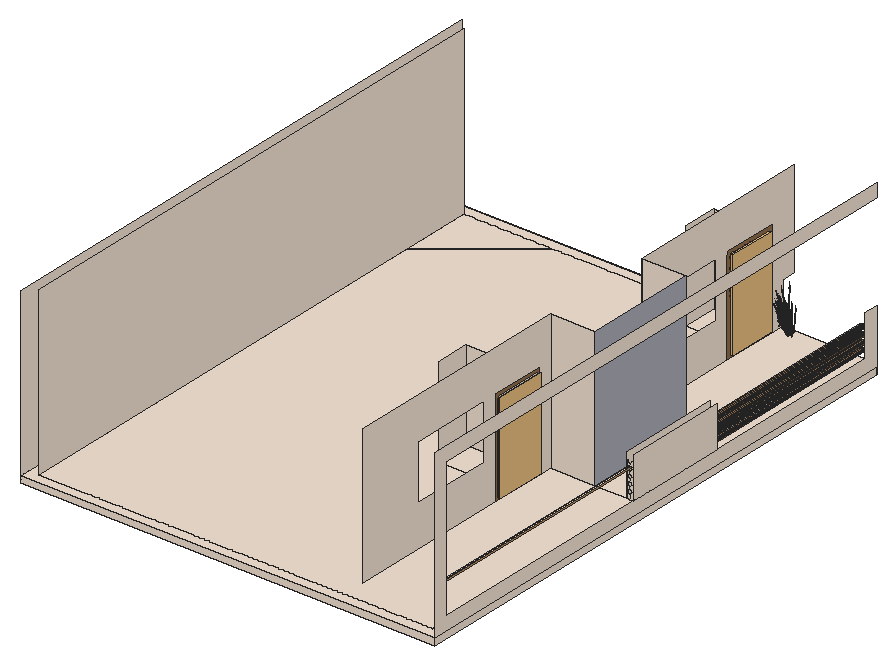
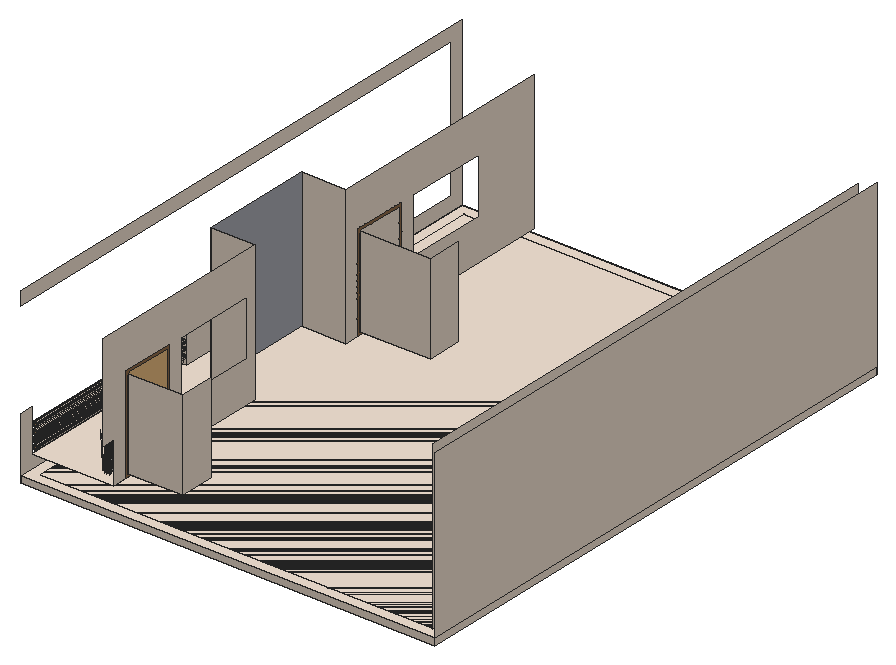
# SketchUp Ruby script. Lengths in inches.
U = 1.inch
M = Sketchup.active_model
def pt(a) = Geom::Point3d.new(a.map { |v| v * U })
def face(e, loops, mat)
  f = e.add_face(loops[0].map { |a| pt(a) })
  loops[1..].each { |l| e.add_face(l.map { |a| pt(a) }).erase! }
  f.material = f.back_material = mat if mat
  f
end
# faces: each face lists its corners as indices into pts; further lists are holes
def faces(e, pts, list, mat = nil) = list.each { |f| face(e, (f[0].is_a?(Array) ? f : [f]).map { |l| l.map { |i| pts[i] } }, mat) }
# xy, xz, yz: faces in a plane at the given z, y or x. An outline is a flat list of corners, or four numbers for a rectangle; further outlines are holes
def ring(l) = l.size == 4 ? [[l[0], l[1]], [l[2], l[1]], [l[2], l[3]], [l[0], l[3]]] : l.each_slice(2).to_a
def flat(e, list, mat, &to3) = list.each { |f| face(e, (f[0].is_a?(Array) ? f : [f]).map { |l| ring(l).map { |u, v| to3.(u, v) } }, mat) }
def xy(e, z, list, mat = nil) = flat(e, list, mat) { |x, y| [x, y, z] }
def xz(e, y, list, mat = nil) = flat(e, list, mat) { |x, z| [x, y, z] }
def yz(e, x, list, mat = nil) = flat(e, list, mat) { |y, z| [x, y, z] }
def lines(e, pts, list) = list.each { |a, b| e.add_line(pt(pts[a]), pt(pts[b])) }
# prism: a flat outline (further loops are holes) pulled along v
def prism(e, loops, v, mat = nil)
  f = face(e, loops, mat); d = Geom::Vector3d.new(v.map { |x| x * U })
  f.pushpull(f.normal.samedirection?(d) ? d.length : -d.length)
end
def box(e, o, s, mat = nil) = prism(e, [[o, [o[0] + s[0], o[1], o[2]], [o[0] + s[0], o[1] + s[1], o[2]], [o[0], o[1] + s[1], o[2]]]], [0, 0, s[2]], mat)
def at(x, y, z, deg = 0) = Geom::Transformation.translation(pt([x, y, z])) * Geom::Transformation.rotation(ORIGIN, Z_AXIS, deg.degrees)
def axes(o, x, y, z) = Geom::Transformation.new([*x, 0, *y, 0, *z, 0, *pt(o).to_a, 1])
def part(name) = M.definitions.add(name)
# library, detail: a bought-in or finely detailed component or shape, given as its bounding box
def library(name, o, s) = part(name).tap { |d| box(d.entities, o, s) }
def detail(e, o, s) = box(e.add_group.entities, o, s)
def put(e, d, t, mat = nil) = e.add_instance(d, t).tap { |i| i.material = mat if mat }
def group(e, t, mat = nil) = e.add_group.tap { |g| g.transformation = t; g.material = mat if mat }.entities
root = M.entities
M.materials.add("C01_Vanilla_Cream").color = [244, 228, 212]
M.materials.add("LightPink_Translucent").color = [144, 107, 117]
M.materials["LightPink_Translucent"].alpha = 0.75
M.materials.add("Marble_20_1K").color = [172, 173, 182]
M.materials.add("Wood_Floor_01_1K").color = [146, 111, 76]
c1 = library("porta+4",[0.2,-5.42,1.33],[46.55,4.72,83.21])
c2 = part("Group\#10")
box(c2.entities,[0,0,0],[360,480,6])
c3 = part("blade")
p = [[2.15,0.21,22],[0,0.17,0],[0.09,0.45,0],[2.18,0.31,22],[2.29,0.31,22],[0.38,0.45,0],
  [2.48,0.24,33],[2.49,0.24,33],[2.48,0.22,33]]
faces(c3.entities,p,[[0,1,2,3],[4,5,2,3],[6,3,4,7],[8,0,3,6]])
c4 = part("seeds")
p = [[0.3,-0.1,1.38],[-0.01,-0.03,1.59],[-0.01,-0.03,0.03],[0.14,-0.07,-0.07],[0.29,-0.03,3],[0.15,0.01,3.11]]
faces(c4.entities,p,[[0,1,2,3],[1,0,4,5]],"LightPink_Translucent")
c5 = part("blade with seeds")
put(c5.entities,c3,at(0,0,0))
put(c5.entities,c4,axes([2.4,0.25,30.99],[1.5799,-0.05474,1.17369],[-0.12525,1.92788,0.29478],[-0.07173,-0.02425,1.56792]))
xy(root,444,[[[0,0,360,480],[9,9,351,471]]],"C01_Vanilla_Cream")
xy(root,450,[[[0,0,360,480],[9,9,351,471]],[9,9,351,471]],"C01_Vanilla_Cream")
xy(root,462,[[326.85,216,354,216,354,306.76,360,306.76,360,468,288,468,288,314.71,326.85,314.71],[354,216,360,306.76]],"C01_Vanilla_Cream")
xy(root,465,[[226.53,171,288,201],[240,423,288,453]],"C01_Vanilla_Cream")
xz(root,201,[[226.53,465,288,543]],"C01_Vanilla_Cream")
xz(root,216,[[288,462,326.85,582],[354,462,357,462,357,466,356.48,466.07,356,466.27,355.59,466.59,355.27,467,355.07,467.48,355,468,354,468],[357,462,360,462,360,468,359,468,358.93,467.48,358.73,467,358.41,466.59,358,466.27,357.52,466.07,357,466],[354,468,355,468,355.07,468.52,355.27,469,355.59,469.41,356,469.73,356.48,469.93,357,470,357,472,356.48,472.07,356,472.27,355.59,472.59,355.27,473,355.07,473.48,355,474,354,474],[359,468,360,468,360,474,359,474,358.93,473.48,358.73,473,358.41,472.59,358,472.27,357.52,472.07,357,472,357,470,357.52,469.93,358,469.73,358.41,469.41,358.73,469,358.93,468.52],
  [354,474,355,474,355.07,474.52,355.27,475,355.59,475.41,356,475.73,356.48,475.93,357,476,357,478,356.48,478.07,356,478.27,355.59,478.59,355.27,479,355.07,479.48,355,480,354,480],[359,474,360,474,360,480,359,480,358.93,479.48,358.73,479,358.41,478.59,358,478.27,357.52,478.07,357,478,357,476,357.52,475.93,358,475.73,358.41,475.41,358.73,475,358.93,474.52],[354,480,355,480,355.07,480.52,355.27,481,355.59,481.41,356,481.73,356.48,481.93,357,482,357,484,356.48,484.07,356,484.27,355.59,484.59,355.27,485,355.07,485.48,355,486,354,486],[359,480,360,480,360,486,359,486,358.93,485.48,358.73,485,358.41,484.59,358,484.27,357.52,484.07,357,484,357,482,357.52,481.93,358,481.73,358.41,481.41,358.73,481,358.93,480.52],[354,486,355,486,355.07,486.52,355.27,487,355.59,487.41,356,487.73,356.48,487.93,357,488,357,490,356.48,490.07,356,490.27,355.59,490.59,355.27,491,355.07,491.48,355,492,354,492],
  [359,486,360,486,360,492,359,492,358.93,491.48,358.73,491,358.41,490.59,358,490.27,357.52,490.07,357,490,357,488,357.52,487.93,358,487.73,358.41,487.41,358.73,487,358.93,486.52]],"C01_Vanilla_Cream")
xz(root,306.76,[[354,462,354,468,355,468,355.07,467.48,355.27,467,355.59,466.59,356,466.27,356.48,466.07,357,466,357,462],[357,462,357,466,357.52,466.07,358,466.27,358.41,466.59,358.73,467,358.93,467.48,359,468,360,468,360,462],[354,468,354,474,355,474,355.07,473.48,355.27,473,355.59,472.59,356,472.27,356.48,472.07,357,472,357,470,356.48,469.93,356,469.73,355.59,469.41,355.27,469,355.07,468.52,355,468],[359,468,358.93,468.52,358.73,469,358.41,469.41,358,469.73,357.52,469.93,357,470,357,472,357.52,472.07,358,472.27,358.41,472.59,358.73,473,358.93,473.48,359,474,360,474,360,468],[354,474,354,480,355,480,355.07,479.48,355.27,479,355.59,478.59,356,478.27,356.48,478.07,357,478,357,476,356.48,475.93,356,475.73,355.59,475.41,355.27,475,355.07,474.52,355,474],
  [359,474,358.93,474.52,358.73,475,358.41,475.41,358,475.73,357.52,475.93,357,476,357,478,357.52,478.07,358,478.27,358.41,478.59,358.73,479,358.93,479.48,359,480,360,480,360,474],[354,480,354,486,355,486,355.07,485.48,355.27,485,355.59,484.59,356,484.27,356.48,484.07,357,484,357,482,356.48,481.93,356,481.73,355.59,481.41,355.27,481,355.07,480.52,355,480],[359,480,358.93,480.52,358.73,481,358.41,481.41,358,481.73,357.52,481.93,357,482,357,484,357.52,484.07,358,484.27,358.41,484.59,358.73,485,358.93,485.48,359,486,360,486,360,480],[354,486,354,492,355,492,355.07,491.48,355.27,491,355.59,490.59,356,490.27,356.48,490.07,357,490,357,488,356.48,487.93,356,487.73,355.59,487.41,355.27,487,355.07,486.52,355,486],[359,486,358.93,486.52,358.73,487,358.41,487.41,358,487.73,357.52,487.93,357,488,357,490,357.52,490.07,358,490.27,358.41,490.59,358.73,491,358.93,491.48,359,492,360,492,360,486]],"C01_Vanilla_Cream")
xz(root,314.71,[[288,462,326.85,582]],"C01_Vanilla_Cream")
xz(root,453,[[240,465,288,543]],"C01_Vanilla_Cream")
yz(root,0,[[0,450,480,594]],"C01_Vanilla_Cream")
yz(root,9,[[9,450,471,594]],"C01_Vanilla_Cream")
yz(root,226.53,[[171,465,201,543]],"C01_Vanilla_Cream")
yz(root,240,[[423,465,453,543]],"C01_Vanilla_Cream")
yz(root,288,[[[12,462,156,462,156,546,204,546,204,462,216,462,216,582,12,582],[72,498,144,546]],[[314.71,462,408,462,408,546,456,546,456,462,468,462,468,498,480,498,480,582,314.71,582],[324,498,396,546]],[159,465,201,543],[411,465,453,543]],"C01_Vanilla_Cream")
yz(root,288,[[[156,462,204,546],[159,465,201,543]],[[408,462,456,546],[411,465,453,543]]],"Wood_Floor_01_1K")
yz(root,326.85,[[216,462,314.71,582]],"Marble_20_1K")
yz(root,354,[[216,462,306.76,498]],"C01_Vanilla_Cream")
yz(root,360,[[0,450,480,450,480,498,468,498,468,462,12,462,12,582,480,582,480,594,0,594],[216,462,306.76,498]],"C01_Vanilla_Cream")
p = [[357,306.76,466],[356.48,306.76,466.07],[356.48,468,466.07],[357,468,466],[357.52,306.76,466.07],[357.52,468,466.07],
  [356,306.76,466.27],[356,468,466.27],[358,306.76,466.27],[358,468,466.27],[355.59,306.76,466.59],[355.59,468,466.59],
  [358.41,306.76,466.59],[358.41,468,466.59],[355.27,306.76,467],[355.27,468,467],[358.73,306.76,467],[358.73,468,467],
  [355.07,306.76,467.48],[355.07,468,467.48],[358.93,306.76,467.48],[358.93,468,467.48],[355,306.76,468],[355,468,468],
  [359,306.76,468],[359,468,468],[355.07,306.76,468.52],[355.07,468,468.52],[358.93,306.76,468.52],[358.93,468,468.52],
  [355.27,306.76,469],[355.27,468,469],[358.73,306.76,469],[358.73,468,469],[355.59,306.76,469.41],[355.59,468,469.41],
  [358.41,306.76,469.41],[358.41,468,469.41],[356,306.76,469.73],[356,468,469.73],[358,306.76,469.73],[358,468,469.73],
  [356.48,306.76,469.93],[356.48,468,469.93],[357.52,306.76,469.93],[357.52,468,469.93],[357,306.76,470],[357,468,470],
  [357,306.76,472],[356.48,306.76,472.07],[356.48,468,472.07],[357,468,472],[357.52,306.76,472.07],[357.52,468,472.07],
  [356,306.76,472.27],[356,468,472.27],[358,306.76,472.27],[358,468,472.27],[355.59,306.76,472.59],[355.59,468,472.59],
  [358.41,306.76,472.59],[358.41,468,472.59],[355.27,306.76,473],[355.27,468,473],[358.73,306.76,473],[358.73,468,473],
  [355.07,306.76,473.48],[355.07,468,473.48],[358.93,306.76,473.48],[358.93,468,473.48],[355,306.76,474],[355,468,474],
  [359,306.76,474],[359,468,474],[355.07,306.76,474.52],[355.07,468,474.52],[358.93,306.76,474.52],[358.93,468,474.52],
  [355.27,306.76,475],[355.27,468,475],[358.73,306.76,475],[358.73,468,475],[355.59,306.76,475.41],[355.59,468,475.41],
  [358.41,306.76,475.41],[358.41,468,475.41],[356,306.76,475.73],[356,468,475.73],[358,306.76,475.73],[358,468,475.73],
  [356.48,306.76,475.93],[356.48,468,475.93],[357.52,306.76,475.93],[357.52,468,475.93],[357,306.76,476],[357,468,476],
  [357,306.76,478],[356.48,306.76,478.07],[356.48,468,478.07],[357,468,478],[357.52,306.76,478.07],[357.52,468,478.07],
  [356,306.76,478.27],[356,468,478.27],[358,306.76,478.27],[358,468,478.27],[355.59,306.76,478.59],[355.59,468,478.59],
  [358.41,306.76,478.59],[358.41,468,478.59],[355.27,306.76,479],[355.27,468,479],[358.73,306.76,479],[358.73,468,479],
  [355.07,306.76,479.48],[355.07,468,479.48],[358.93,306.76,479.48],[358.93,468,479.48],[355,306.76,480],[355,468,480],
  [359,306.76,480],[359,468,480],[355.07,306.76,480.52],[355.07,468,480.52],[358.93,306.76,480.52],[358.93,468,480.52],
  [355.27,306.76,481],[355.27,468,481],[358.73,306.76,481],[358.73,468,481],[355.59,306.76,481.41],[355.59,468,481.41],
  [358.41,306.76,481.41],[358.41,468,481.41],[356,306.76,481.73],[356,468,481.73],[358,306.76,481.73],[358,468,481.73],
  [356.48,306.76,481.93],[356.48,468,481.93],[357.52,306.76,481.93],[357.52,468,481.93],[357,306.76,482],[357,468,482],
  [357,306.76,484],[356.48,306.76,484.07],[356.48,468,484.07],[357,468,484],[357.52,306.76,484.07],[357.52,468,484.07],
  [356,306.76,484.27],[356,468,484.27],[358,306.76,484.27],[358,468,484.27],[355.59,306.76,484.59],[355.59,468,484.59],
  [358.41,306.76,484.59],[358.41,468,484.59],[355.27,306.76,485],[355.27,468,485],[358.73,306.76,485],[358.73,468,485],
  [355.07,306.76,485.48],[355.07,468,485.48],[358.93,306.76,485.48],[358.93,468,485.48],[355,306.76,486],[355,468,486],
  [359,306.76,486],[359,468,486],[355.07,306.76,486.52],[355.07,468,486.52],[358.93,306.76,486.52],[358.93,468,486.52],
  [355.27,306.76,487],[355.27,468,487],[358.73,306.76,487],[358.73,468,487],[355.59,306.76,487.41],[355.59,468,487.41],
  [358.41,306.76,487.41],[358.41,468,487.41],[358.41,216,487.41],[358,216,487.73],[358,12,487.73],[358.41,12,487.41],
  [356,306.76,487.73],[356,468,487.73],[358,306.76,487.73],[358,468,487.73],[356.48,216,487.93],[356,216,487.73],
  [356,12,487.73],[356.48,12,487.93],[357.52,216,487.93],[357.52,12,487.93],[356.48,306.76,487.93],[356.48,468,487.93],
  [357.52,306.76,487.93],[357.52,468,487.93],[357,306.76,488],[357,468,488]]
faces(root,p,[[0,1,2,3],[1,6,7,2],[6,10,11,7],[10,14,15,11],[14,18,19,15],[18,22,23,19],[22,26,27,23],[26,30,31,27],
  [30,34,35,31],[34,38,39,35],[38,42,43,39],[42,46,47,43],[48,49,50,51],[49,54,55,50],[54,58,59,55],[58,62,63,59],
  [62,66,67,63],[66,70,71,67],[70,74,75,71],[74,78,79,75],[78,82,83,79],[82,86,87,83],[86,90,91,87],[90,94,95,91],
  [96,97,98,99],[97,102,103,98],[102,106,107,103],[106,110,111,107],[110,114,115,111],[114,118,119,115],[118,122,123,119],[122,126,127,123],
  [126,130,131,127],[130,134,135,131],[134,138,139,135],[138,142,143,139],[144,145,146,147],[145,150,151,146],[150,154,155,151],[154,158,159,155],
  [158,162,163,159],[162,166,167,163],[166,170,171,167],[170,174,175,171],[174,178,179,175],[178,186,187,179],[190,191,192,193],[186,196,197,187],
  [196,200,201,197]],"C01_Vanilla_Cream")
faces(root,p,[[4,0,3,5],[8,4,5,9],[12,8,9,13],[16,12,13,17],[20,16,17,21],[24,20,21,25],[28,24,25,29],[32,28,29,33],
  [36,32,33,37],[40,36,37,41],[44,40,41,45],[46,44,45,47],[52,48,51,53],[56,52,53,57],[60,56,57,61],[64,60,61,65],
  [68,64,65,69],[72,68,69,73],[76,72,73,77],[80,76,77,81],[84,80,81,85],[88,84,85,89],[92,88,89,93],[94,92,93,95],
  [100,96,99,101],[104,100,101,105],[108,104,105,109],[112,108,109,113],[116,112,113,117],[120,116,117,121],[124,120,121,125],[128,124,125,129],
  [132,128,129,133],[136,132,133,137],[140,136,137,141],[142,140,141,143],[148,144,147,149],[152,148,149,153],[156,152,153,157],[160,156,157,161],
  [164,160,161,165],[168,164,165,169],[172,168,169,173],[176,172,173,177],[180,176,177,181],[182,183,184,185],[188,180,181,189],[183,194,195,184],
  [198,188,189,199],[200,198,199,201]],"Wood_Floor_01_1K")
put(root,c1,axes([289.83,157.29,463.73],[0,0.9504,0],[-0.24166,0,0],[0,0,0.9416]),"C01_Vanilla_Cream")
put(root,c2,at(0,0,444),"C01_Vanilla_Cream")
put(root,c1,axes([291.16,410.82,463.74],[0,0.8978,0],[0.58403,0,0],[0,0,0.94]),"C01_Vanilla_Cream")
put(root,c5,axes([300,459.19,464.91],[0.12726,0.15818,1.28532],[-0.58807,0.13317,0.10393],[-0.13291,-0.24832,0.54946]))
put(root,c5,axes([300.97,458.14,465.54],[-0.08515,-0.06907,1.31208],[-0.56828,0.04379,-0.2075],[-0.0907,-0.16522,0.10523]))
put(root,c5,axes([302.29,458.96,463.94],[-0.15825,0.09972,1.07251],[-0.47395,-0.17454,-0.23066],[0.08785,-0.21706,0.45856]))
put(root,c5,axes([301.57,459.3,465.74],[-0.26572,-0.40059,-0.53284],[0.54698,-0.22325,0.0643],[-0.06214,-0.19355,0.75375]))
put(root,c5,axes([299.84,458.77,463.94],[-0.03371,0.16116,1.07251],[-0.49286,0.13491,-0.23066],[-0.11521,-0.20831,0.45856]))
put(root,c5,axes([301.11,458.41,463.12],[-0.09338,0.01775,1.32257],[-0.51641,-0.1998,-0.20205],[0.00867,-0.16666,0.22528]))
put(root,c5,axes([302.67,459.7,465.74],[0.01449,-0.45571,-0.53284],[0.61002,0.03061,0.0643],[0.06438,-0.19306,0.75375]))
put(root,c5,axes([303.52,458.98,465.54],[-0.00537,-0.09805,1.31208],[-0.45391,-0.28338,-0.2075],[0.07018,-0.17178,0.10523]))
put(root,c5,axes([301.62,458.96,465.39],[0.16784,-0.37886,-0.2656],[0.48968,0.1105,0.3429],[-0.0449,-0.15254,0.65611]))
put(root,c5,axes([301.99,459.46,464.91],[-0.10366,0.16934,1.28532],[-0.43488,-0.35044,0.10393],[0.19618,-0.21841,0.54946]))
put(root,c5,axes([303.4,458.63,465.53],[-0.05654,0.03763,1.33037],[-0.55396,-0.12696,-0.12571],[-0.02005,-0.16422,0.23543]))
put(root,c5,axes([301.37,459.22,465.51],[-0.54728,-0.1235,-0.38324],[0.18759,-0.42344,-0.29685],[-0.05018,-0.17048,0.7333]))
put(root,c5,axes([301.71,458.16,464.07],[0.07142,0.28728,0.86145],[-0.3962,-0.15911,0.63294],[0.04263,-0.1471,0.18974]))
put(root,c5,axes([302.55,459.54,465.51],[-0.39855,-0.33102,-0.38324],[0.42102,-0.2899,-0.29685],[0.06064,-0.16819,0.7333]))
put(root,c5,axes([300.39,457.91,465.53],[-0.01039,0.05905,1.33037],[-0.51226,0.21431,-0.12571],[-0.15074,-0.10955,0.23543]))
put(root,c5,axes([300.28,458.96,465.82],[0.62019,-0.12663,0.40322],[0.10763,0.49673,0.33247],[-0.14586,-0.1464,0.83437]))
put(root,c5,axes([301.68,459.05,465.55],[0.54859,0.1288,0.36002],[-0.18759,0.42344,0.29685],[-0.03297,-0.16652,0.74497]))
put(root,c5,axes([301.84,459.2,465.78],[-0.54481,0.22937,-0.0912],[-0.26773,-0.4071,-0.50621],[-0.07188,-0.17155,0.76918]))
put(root,c5,axes([302.97,459.72,465.78],[-0.61188,-0.02441,-0.0912],[0.01672,-0.46217,-0.50621],[0.0425,-0.178,0.76918]))
put(root,c5,axes([302.92,459.42,465.39],[0.3767,-0.25939,-0.2656],[0.3566,0.29618,0.3429],[0.05426,-0.15048,0.65611]))
put(root,c5,axes([299.67,458.51,464.07],[0.29042,0.17147,0.86145],[-0.42295,0.10307,0.63294],[-0.0905,-0.13178,0.18974]))
put(root,c5,axes([301.82,459.02,465.55],[0.41024,-0.16744,0.04823],[0.2008,0.30532,0.37966],[-0.03962,-0.13459,0.57892]))
put(root,c5,axes([300.37,459.42,465.74],[-0.47473,-0.23813,-0.53284],[0.33738,-0.41728,0.0643],[-0.172,-0.14218,0.75375]))
put(root,c5,axes([300.21,459.1,465.39],[-0.08599,-0.39682,-0.2656],[0.49155,-0.10478,0.3429],[-0.13203,-0.11372,0.65611]))
put(root,c5,axes([300.42,459.07,465.55],[0.25304,-0.31296,0.04823],[0.36033,0.18221,0.37966],[-0.11649,-0.10034,0.57892]))
put(root,c5,axes([299.4375,459.02,463.12],[-0.05393,0.0649,1.32257],[-0.545,0.13993,-0.20205],[-0.13166,-0.12729,0.22528]))
put(root,c5,axes([300.34,460.81,463.57],[-0.22864,-0.5052,-0.52377],[0.65862,-0.18195,-0.13747],[-0.02527,-0.17107,1.15612]))
put(root,c5,axes([299.15,459.68,464.91],[0.2068,0.08488,1.28532],[-0.42797,0.35609,0.10393],[-0.26673,-0.16064,0.54946]))
put(root,c5,axes([303.39,459.26,463.12],[-0.08333,-0.03881,1.32257],[-0.21404,-0.4336,-0.20205],[0.14439,-0.11767,0.22528]))
put(root,c5,axes([301.67,459.36,465.79],[-0.16784,0.37886,0.2656],[-0.48968,-0.1105,-0.3429],[-0.0449,-0.15254,0.65611]))
put(root,c5,axes([300.15,459.43,465.51],[-0.54938,0.11711,-0.38324],[-0.0961,-0.44351,-0.29685],[-0.14756,-0.1271,0.7333]))
put(root,c5,axes([302.92,459.52,465.55],[0.39645,0.33614,0.36002],[-0.42102,0.2899,0.29685],[0.07313,-0.15771,0.74497]))
put(root,c5,axes([300.53,459.03,466.07],[-0.37157,0.4723,-0.10215],[-0.5381,-0.2721,-0.56695],[-0.18705,-0.13344,0.86148]))
put(root,c5,axes([303.07,459.55,465.55],[0.45752,0.02296,0.04823],[-0.01254,0.34663,0.37966],[0.04787,-0.13278,0.57892]))
put(root,c5,axes([302.73,459.79,465.79],[-0.3767,0.25939,0.2656],[-0.3566,-0.29618,-0.3429],[0.05426,-0.15048,0.65611]))
put(root,c5,axes([303.39,460.49,465.74],[0.29081,-0.38873,-0.53284],[0.5096,0.27626,0.0643],[0.17364,-0.14084,0.75375]))
put(root,c5,axes([300.25,459.36,463.78],[-0.34808,-0.49367,0],[0.58235,-0.27531,-0.38706],[0.13264,-0.0627,1.22783]))
